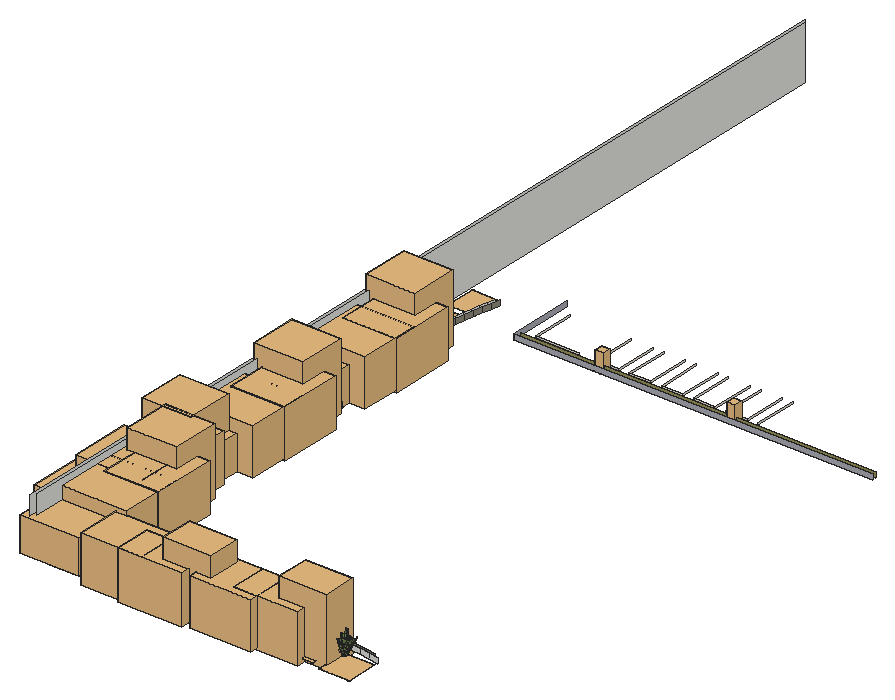
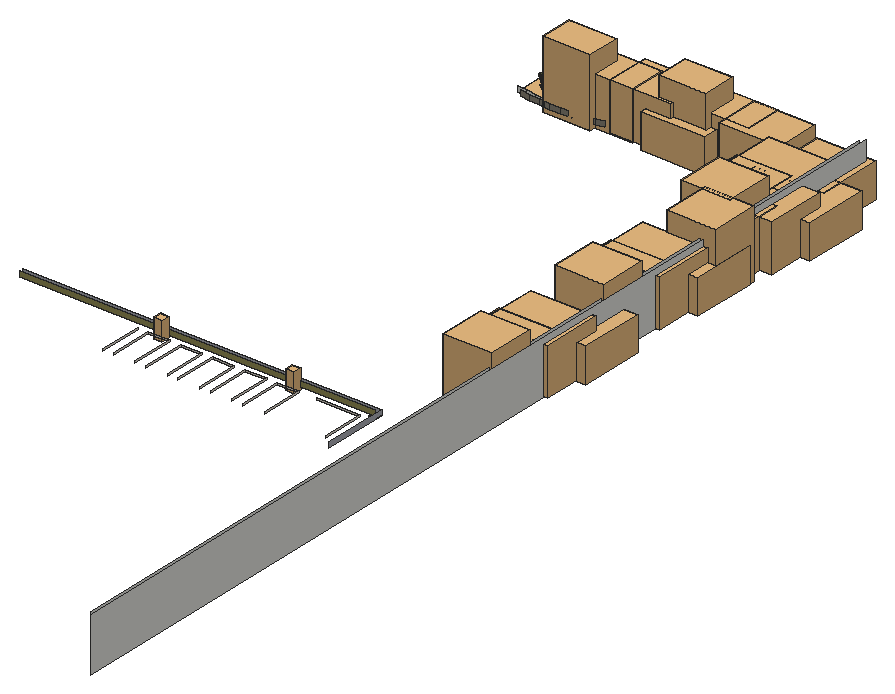
# SketchUp Ruby script. Lengths in inches.
U = 1.inch
M = Sketchup.active_model
def pt(a) = Geom::Point3d.new(a.map { |v| v * U })
def face(e, loops, mat)
  f = e.add_face(loops[0].map { |a| pt(a) })
  loops[1..].each { |l| e.add_face(l.map { |a| pt(a) }).erase! }
  f.material = f.back_material = mat if mat
  f
end
# faces: each face lists its corners as indices into pts; further lists are holes
def faces(e, pts, list, mat = nil) = list.each { |f| face(e, (f[0].is_a?(Array) ? f : [f]).map { |l| l.map { |i| pts[i] } }, mat) }
# xy, xz, yz: faces in a plane at the given z, y or x. An outline is a flat list of corners, or four numbers for a rectangle; further outlines are holes
def ring(l) = l.size == 4 ? [[l[0], l[1]], [l[2], l[1]], [l[2], l[3]], [l[0], l[3]]] : l.each_slice(2).to_a
def flat(e, list, mat, &to3) = list.each { |f| face(e, (f[0].is_a?(Array) ? f : [f]).map { |l| ring(l).map { |u, v| to3.(u, v) } }, mat) }
def xy(e, z, list, mat = nil) = flat(e, list, mat) { |x, y| [x, y, z] }
def xz(e, y, list, mat = nil) = flat(e, list, mat) { |x, z| [x, y, z] }
def yz(e, x, list, mat = nil) = flat(e, list, mat) { |y, z| [x, y, z] }
def lines(e, pts, list) = list.each { |a, b| e.add_line(pt(pts[a]), pt(pts[b])) }
# prism: a flat outline (further loops are holes) pulled along v
def prism(e, loops, v, mat = nil)
  f = face(e, loops, mat); d = Geom::Vector3d.new(v.map { |x| x * U })
  f.pushpull(f.normal.samedirection?(d) ? d.length : -d.length)
end
def box(e, o, s, mat = nil) = prism(e, [[o, [o[0] + s[0], o[1], o[2]], [o[0] + s[0], o[1] + s[1], o[2]], [o[0], o[1] + s[1], o[2]]]], [0, 0, s[2]], mat)
def at(x, y, z, deg = 0) = Geom::Transformation.translation(pt([x, y, z])) * Geom::Transformation.rotation(ORIGIN, Z_AXIS, deg.degrees)
def axes(o, x, y, z) = Geom::Transformation.new([*x, 0, *y, 0, *z, 0, *pt(o).to_a, 1])
def part(name) = M.definitions.add(name)
# library, detail: a bought-in or finely detailed component or shape, given as its bounding box
def library(name, o, s) = part(name).tap { |d| box(d.entities, o, s) }
def detail(e, o, s) = box(e.add_group.entities, o, s)
def put(e, d, t, mat = nil) = e.add_instance(d, t).tap { |i| i.material = mat if mat }
def group(e, t, mat = nil) = e.add_group.tap { |g| g.transformation = t; g.material = mat if mat }.entities
root = M.entities
M.materials.add("Marble_01_1K").color = [230, 221, 211]
M.materials.add("Marble_20_1K").color = [172, 173, 182]
M.materials.add("Material__4").color = [36, 36, 36]
M.materials.add("Material__6").color = [79, 108, 5]
M.materials.add("Plaster_06_1K").color = [141, 135, 122]
M.materials.add("Soil_04_1K").color = [152, 146, 88]
M.materials.add("calathea lutea").color = [121, 145, 80]
c1 = library("ew",[-14.92,-16.84,0],[29.84,33.68,0.01])
c2 = library("t1",[-17.79,-17.21,0],[35.58,34.42,0.01])
c3 = library("tt",[-12.4,-12.1,0],[24.8,24.2,0.01])
c4 = part("Group\#156")
g1 = group(c4.entities,at(8.61,38.85,0))
xy(g1,0,[[0,0,2.82,19.1,22.58,0],[22.58,0,2.82,19.1,22.58,19.1]],"calathea lutea")
p = [[2.82,19.1,0],[7.19,48.22,5.13],[10.77,48.22,5.13],[12.74,48.22,5.13],[22.58,48.22,5.13],[22.58,19.1,0]]
faces(g1,p,[[0,1,2,3,4,5]],"calathea lutea")
g2 = group(c4.entities,at(-0.77,-7.77,0))
p = [[14.8125,23.31,1.46],[21.35,23.31,0],[14.8125,0,1.46],[21.35,0,0],[27.89,0,1.46],[27.89,23.31,1.46],
  [8.27,46.62,2.92],[21.35,46.62,0],[34.4375,46.62,2.92],[4.47,23.31,6.43],[0,0,8.59],[33.76,0,4.28],
  [33.76,23.31,4.28]]
faces(g2,p,[[0,1,2],[3,2,1],[4,3,5],[1,5,3],[6,7,0],[1,0,7],[5,1,8],[7,8,1],
  [9,0,2,10],[11,4,5,12],[9,6,0],[12,5,8]],"calathea lutea")
c5 = part("Group\#150")
xy(c5.entities,0,[[0,0,0,33.87,27.21,33.87,19.71,0]],"calathea lutea")
c6 = part("Group\#157")
xy(c6.entities,1.04,[[21.13,33.87,21.13,57.59,32.375,57.59,27.12,33.87]],"calathea lutea")
xy(c6.entities,1.32,[[0.12,33.87,7.74,57.59]],"calathea lutea")
p = [[7.74,33.87,1.32],[11.8,57.59,0.61],[15.24,57.59,0],[15.24,33.87,0],[18.43,57.59,0.5625],[21.13,57.59,1.04],
  [21.13,33.87,1.04],[15.24,77.7,2.36],[21.13,77.7,3.4],[7.74,57.59,1.32],[7.74,77.7,3.69],[36.83,77.7,3.4],
  [32.375,57.59,1.04],[0.12,57.59,1.32],[0.12,77.7,3.69]]
faces(c6.entities,p,[[0,1,2,3],[3,2,4],[3,4,5,6],[7,2,1],[8,4,2,7],[0,9,1],[7,1,9,10],[8,5,4],
  [11,12,5,8],[10,9,13,14]],"calathea lutea")
put(c6.entities,c5,axes([0,-16.9375,0],[1,0,0],[0,1.5,0],[0,0,1]))
c7 = part("Group\#155")
g3 = group(c7.entities,at(0,-17.3,0))
xy(g3,0,[[0,0,28.07,51.9]],"calathea lutea")
g4 = group(c7.entities,at(0.9,34.6,0))
xy(g4,0,[[13.14,0,13.14,26.22,16.85,26.22],[13.14,0,16.85,26.22,20.16,26.22,20.16,0]],"calathea lutea")
p = [[6.36,0,1.82],[9.95,26.22,0.86],[13.14,26.22,0],[13.14,0,0],[20.16,0,0],[20.16,26.22,0],
  [27.07,26.22,1.22],[27.07,0,1.22],[13.14,49.5625,5.91],[20.16,49.5625,5.91],[16.85,26.22,0],[27.07,49.5625,7.125],
  [6.36,26.22,1.82],[6.36,49.5625,7.72],[0,0,4.78],[0,26.22,4.78],[0,49.5625,10.6875]]
faces(g4,p,[[0,1,2,3],[4,5,6,7],[8,2,1],[9,10,2,8],[9,5,10],[11,6,5,9],[0,12,1],[8,1,12,13],
  [14,15,12,0],[13,12,15,16]],"calathea lutea")
c8 = part("Group\#154")
put(c8.entities,c5,axes([0,-16.9375,0],[1,0,0],[0,1.5,0],[0,0,1]))
g5 = group(c8.entities,at(-0.23,33.4,-0.35))
p = [[15.12,39.14,-19.87],[15.12,20.54,-11.86],[11.68,20.84,-11.33],[21.02,39.66,-18.97],[18.3125,20.82,-11.37],[7.62,21.2,-10.71],
  [7.62,39.8,-18.72],[21.02,21.06,-10.96],[36.72,39.66,-18.97],[32.26,21.06,-10.96],[0,21.2,-10.71],[0,39.8,-18.72],
  [7.62,0.66,1.15],[15.12,0,0],[21.02,0.52,0.9],[27.01,0.52,0.9],[0,0.66,1.15]]
faces(g5,p,[[0,1,2],[3,4,1,0],[0,2,5,6],[3,7,4],[8,9,7,3],[6,5,10,11],[12,2,1,13],[13,1,4],
  [13,4,7,14],[12,5,2],[14,7,9,15],[16,10,5,12]],"calathea lutea")
c9 = part("Foliage cluster")
put(c9.entities,c4,axes([37.24,8.07,75.17],[1,0,0],[0,0.45554,-0.89021],[0,0.89021,0.45554]))
put(c9.entities,c6,axes([69.44,65.48,16.68],[-0.53288,-0.84619,0],[0.14694,-0.09253,0.98481],[-0.83334,0.52478,0.17365]))
put(c9.entities,c7,axes([47.9375,70.43,17.04],[0.74664,-0.66523,0],[0.11552,0.12965,0.98481],[-0.65512,-0.7353,0.17365]))
put(c9.entities,c4,axes([76.19,10.66,75.17],[0.70711,0.70711,0],[-0.32212,0.32212,-0.89021],[-0.62948,0.62948,0.45554]))
put(c9.entities,c4,axes([101.91,40.03,75.17],[0,1,0],[-0.45554,0,-0.89021],[-0.89021,0,0.45554]))
put(c9.entities,c4,axes([99.32,78.99,75.17],[-0.70711,0.70711,0],[-0.32212,-0.32212,-0.89021],[-0.62948,-0.62948,0.45554]))
put(c9.entities,c7,axes([34.81,63.36,17.04],[0.99956,-0.02967,0],[0.00515,0.17357,0.98481],[-0.02922,-0.98437,0.17365]))
put(c9.entities,c7,axes([48,37.4,15.8],[-0.14436,0.98953,0],[-0.40248,-0.05871,0.91355],[0.90398,0.13188,0.40674]))
put(c9.entities,c6,axes([56.87,39.77,12.28],[-0.67695,0.4263,0],[-0.18016,-0.28609,0.72505],[0.38636,0.61353,0.33809]))
put(c9.entities,c6,axes([36.12,43.25,12.28],[0.18947,0.77724,0],[-0.32848,0.08007,0.72505],[0.70442,-0.17172,0.33809]))
put(c9.entities,c8,axes([35.1,54.93,11.375],[0.79719,0.06694,0],[-0.03636,0.43302,0.6717],[0.05621,-0.66934,0.43454]))
put(c9.entities,c6,axes([41.66,47.32,12.28],[0.45082,0.66088,0],[-0.2793,0.19053,0.72505],[0.59896,-0.40858,0.33809]))
put(c9.entities,c6,axes([47.89,59.4,12.28],[0.79719,0.06694,0],[-0.02829,0.33691,0.72505],[0.06067,-0.7225,0.33809]))
put(c9.entities,c8,axes([29.53,49.96,11.375],[0.65692,0.45657,0],[-0.248,0.35682,0.6717],[0.38335,-0.55156,0.43454]))
put(c9.entities,c8,axes([29.9,49.27,12.86],[0.34062,0.72386,0],[-0.22849,0.10752,0.7591],[0.68685,-0.32321,0.25252]))
put(c9.entities,c8,axes([36.33,48.82,8.99],[0.09232,0.62522,0],[-0.3396,0.05015,0.53064],[0.52495,-0.07752,0.34329]))
put(c9.entities,c8,axes([49.82,38.52,8.99],[-0.54622,0.31791,0],[-0.17268,-0.29669,0.53064],[0.26692,0.45862,0.34329]))
put(c9.entities,c8,axes([55.68,39.21,8.99],[-0.632,0.00221,0],[-0.0012,-0.34328,0.53064],[0.00185,0.53064,0.34329]))
c10 = library("Group\#28",[0,0,0],[86.94,78.77,46.4375])
c11 = library("Group\#14",[-978.71,-103.24,719.12],[90.2,76.4,68.29])
c12 = library("Group\#13",[-906.16,-138.28,686.8],[98.25,106.18,75.79])
c13 = library("Group\#202",[-3.47,-2.45,12.47],[53.14,54.93,75.51])
c14 = part("Group\#41")
put(c14.entities,c9,axes([161.54,64.35,6.01],[0.19523,-0.19694,0],[0.19694,0.19523,0],[0,0,0.24957]))
put(c14.entities,c10,axes([0,37.34,0.92],[0.83,0,0],[0,0.83,0],[0,0,0.83]))
put(c14.entities,c11,axes([859.63,98.87,-568.1],[0.79,0,0],[0,0.79,0],[0,0,0.79]),"Material__4")
put(c14.entities,c12,axes([669.69,114.28,-472.48],[0.69,0,0],[0,0.69,0],[0,0,0.69]),"Material__6")
put(c14.entities,c13,at(132.78,33.9375,-12.6))
c15 = library("light",[-4,-4,0],[8,8,0.01])
c16 = library("Group\#54",[0,0,0],[2062.46,2062.46,4833.66])
c17 = part("Landscape+Light")
put(c17.entities,c16,at(-2096.57,-1031.23,-3775.98))
xz(root,562.78,[[98.71,0,498.69,6]],"Marble_20_1K")
xz(root,567.28,[[103.21,0,498.69,6]],"Soil_04_1K")
xz(root,576.64,[[180.08,0,204.08,2],[216.08,0,240.08,2],[252.08,0,276.08,2],[288.08,0,312.08,2],[324.08,0,348.08,2]],"Marble_01_1K")
xz(root,576.78,[[111.43,0,159.43,2]],"Marble_01_1K")
yz(root,8.46,[[0.95,0,1080.74,60]])
yz(root,12.46,[[4.95,0,1076.74,60]])
yz(root,98.71,[[562.78,0,636.6,6]],"Marble_20_1K")
yz(root,111.43,[[576.78,0,624.64,2]],"Marble_01_1K")
yz(root,180.08,[[576.64,0,624.64,2]],"Marble_01_1K")
yz(root,204.08,[[576.64,0,624.64,2]],"Marble_01_1K")
yz(root,216.08,[[576.64,0,624.64,2]],"Marble_01_1K")
yz(root,240.08,[[576.64,0,624.64,2]],"Marble_01_1K")
yz(root,252.08,[[576.64,0,624.64,2]],"Marble_01_1K")
yz(root,276.08,[[576.64,0,624.64,2]],"Marble_01_1K")
yz(root,288.08,[[576.64,0,624.64,2]],"Marble_01_1K")
yz(root,312.08,[[576.64,0,624.64,2]],"Marble_01_1K")
yz(root,324.08,[[576.64,0,624.64,2]],"Marble_01_1K")
yz(root,348.08,[[576.64,0,624.64,2]],"Marble_01_1K")
yz(root,360.08,[[576.64,0,624.64,2]],"Marble_01_1K")
p = [[183.9,25.07,0],[194.74,24.51,0],[194.74,24.51,6],[183.9,25.07,6],[205.71,25.03,0],[205.71,25.03,6],
  [216.79,26.42,0],[216.79,26.42,6],[173.26,26.9,0],[173.26,26.9,6],[227.98,28.46,0],[227.98,28.46,6],
  [162.9,29.8,0],[162.9,29.8,6],[195.48,27.51,0],[184.7,28,0],[184.7,28,6],[195.48,27.51,6],
  [206.47,28.12,0],[206.47,28.12,6],[174.14,29.78,0],[174.14,29.78,6],[217.65,29.59,0],[217.65,29.59,6],
  [239.25,30.9375,0],[239.25,30.9375,6],[229,31.73,0],[229,31.73,6],[152.68,33.2,0],[152.68,33.2,6],
  [163.75,32.68,0],[163.75,32.68,6],[250.61,33.66,0],[250.61,33.66,6],[240.5,34.3125,0],[240.5,34.3125,6],
  [153.33,36.15,0],[153.33,36.15,6],[36.37,33.08,0],[45.35,34.71,0],[45.35,34.71,6],[36.37,33.08,6],
  [37.51,35.49,0],[37.51,35.49,6],[142.43,36.56,0],[142.43,36.56,6],[262.02,36.42,0],[262.02,36.42,6],
  [252.13,37.12,0],[252.13,37.12,6],[54.59,36.375,0],[54.59,36.375,6],[38.66,37.9,0],[38.66,37.9,6],
  [142.71,39.61,0],[142.71,39.61,6],[64.7,38.09,0],[64.7,38.09,6],[273.48,39.01,0],[273.48,39.01,6],
  [131.97,39.34,0],[131.97,39.34,6],[51.57,38.89,0],[41.67,37.13,0],[41.67,37.13,6],[51.57,38.89,6],
  [43.09,40.39,0],[43.09,40.39,6],[263.875,39.93,0],[263.875,39.93,6],[39.81,40.34,0],[39.81,40.34,6],
  [75.5,39.68,0],[75.5,39.68,6],[61.79,40.65,0],[61.79,40.65,6],[284.95,41.24,0],[284.95,41.24,6],
  [121.11,41.12,0],[121.11,41.12,6],[354.15,41.14,0],[365.76,39.31,0],[365.76,39.31,6],[354.15,41.14,6],
  [131.72,42.47,0],[131.72,42.47,6],[86.77,40.96,0],[86.77,40.96,6],[275.71,42.54,0],[275.71,42.54,6],
  [41,43.32,0],[41,43.32,6],[44.54,44.33,0],[44.54,44.33,6],[72.8,42.34,0],[72.8,42.34,6],
  [98.28,41.75,0],[98.28,41.75,6],[109.81,41.86,0],[109.81,41.86,6],[342.54,42.61,0],[342.54,42.61,6],
  [296.43,42.92,0],[296.43,42.92,6],[84.39,43.75,0],[84.39,43.75,6],[120.22,44.23,0],[120.22,44.23,6],
  [287.6,44.73,0],[287.6,44.73,6],[330.96,43.62,0],[330.96,43.62,6],[307.9,43.87,0],[307.9,43.87,6],
  [42.25,47.02,0],[42.25,47.02,6],[359.53,43.37,0],[347.53,45.05,0],[347.53,45.05,6],[359.53,43.37,6],
  [319.41,44.07,0],[319.41,44.07,6],[96.32,44.66,0],[96.32,44.66,6],[108.34,44.89,0],[108.34,44.89,6],
  [46,49.13,0],[46,49.13,6],[299.55,46.27,0],[299.55,46.27,6],[335.52,46.29,0],[335.52,46.29,6],
  [311.53,47.01,0],[311.53,47.01,6],[323.52,46.98,0],[323.52,46.98,6],[43.53,51.45,0],[43.53,51.45,6],
  [47.49,54.8125,0],[47.49,54.8125,6],[44.84,56.61,0],[44.84,56.61,6],[48.99,61.4,0],[48.99,61.4,6],
  [46.16,62.5,0],[46.16,62.5,6],[50.52,68.9,0],[50.52,68.9,6],[47.51,69.13,0],[47.51,69.13,6],
  [52.08,77.33,0],[52.08,77.33,6],[48.88,76.51,0],[48.88,76.51,6],[50.3125,84.62,0],[50.3125,84.62,6],
  [53.7,86.63,0],[53.7,86.63,6],[51.73,93.31,0],[51.73,93.31,6],[55.27,96.65,0],[55.27,96.65,6],
  [53.03,102.4375,0],[53.03,102.4375,6],[56.63,107.19,0],[56.63,107.19,6],[54.11,111.88,0],[54.11,111.88,6],
  [57.64,118.07,0],[57.64,118.07,6],[54.85,121.51,0],[54.85,121.51,6],[58.12,129.1,0],[58.12,129.1,6],
  [55.14,131.18,0],[55.14,131.18,6],[57.92,140.1,0],[57.92,140.1,6],[54.88,140.77,0],[54.88,140.77,6],
  [56.89,150.88,0],[56.89,150.88,6],[53.96,150.125,0],[53.96,150.125,6],[52.3,159.14,0],[52.3,159.14,6],
  [54.875,161.27,0],[54.875,161.27,6],[49.9375,167.89,0],[49.9375,167.89,6],[52.04,171.24,0],[52.04,171.24,6],
  [47.16,176.49,0],[47.16,176.49,6],[48.82,180.9375,0],[48.82,180.9375,6],[44.27,185.04,0],[44.27,185.04,6],
  [45.66,190.49,0],[45.66,190.49,6],[41.59,193.65,0],[41.59,193.65,6],[43.02,200.04,0],[43.02,200.04,6],
  [39.4375,202.41,0],[39.4375,202.41,6],[41.33,209.72,0],[41.33,209.72,6],[38.14,211.375,0],[38.14,211.375,6],
  [40.74,219.59,0],[40.74,219.59,6],[37.73,220.46,0],[37.73,220.46,6],[41.1,229.64,0],[41.1,229.64,6],
  [38.09,229.64,0],[38.09,229.64,6],[39.08,238.9,0],[39.08,238.9,6],[42.24,239.85,0],[42.24,239.85,6],
  [40.58,248.23,0],[40.58,248.23,6],[44,250.22,0],[44,250.22,6],[42.46,257.64,0],[42.46,257.64,6],
  [46.21,260.72,0],[46.21,260.72,6],[44.61,267.1,0],[44.61,267.1,6],[48.7,271.34,0],[48.7,271.34,6],
  [46.9,276.62,0],[46.9,276.62,6],[51.3,282.06,0],[51.3,282.06,6],[49.21,286.18,0],[49.21,286.18,6],
  [53.86,292.86,0],[53.86,292.86,6],[51.43,295.76,0],[51.43,295.76,6],[56.18,303.74,0],[56.18,303.74,6],
  [53.45,305.375,0],[53.45,305.375,6],[58.125,314.67,0],[58.125,314.67,6],[55.14,314.99,0],[55.14,314.99,6],
  [59.51,325.64,0],[59.51,325.64,6],[56.39,324.6,0],[56.39,324.6,6],[57.11,334.21,0],[57.11,334.21,6],
  [60.21,336.63,0],[60.21,336.63,6],[57.31,343.85,0],[57.31,343.85,6],[60.26,347.64,0],[60.26,347.64,6],
  [57.04,353.52,0],[57.04,353.52,6],[59.73,358.66,0],[59.73,358.66,6],[56.36,363.22,0],[56.36,363.22,6],
  [58.73,369.68,0],[58.73,369.68,6],[55.33,372.93,0],[55.33,372.93,6],[57.3125,380.7,0],[57.3125,380.7,6],
  [53.99,382.65,0],[53.99,382.65,6],[55.58,391.71,0],[55.58,391.71,6],[52.42,392.38,0],[52.42,392.38,6],
  [53.61,402.7,0],[53.61,402.7,6],[50.66,402.12,0],[50.66,402.12,6],[48.78,411.85,0],[48.78,411.85,6],
  [51.48,413.66,0],[51.48,413.66,6],[46.83,421.58,0],[46.83,421.58,6],[49.28,424.6,0],[49.28,424.6,6],
  [44.87,431.29,0],[44.87,431.29,6],[47.09,435.5,0],[47.09,435.5,6],[42.96,440.99,0],[42.96,440.99,6],
  [45,446.36,0],[45,446.36,6],[41.16,450.67,0],[41.16,450.67,6],[43.08,457.16,0],[43.08,457.16,6],
  [39.52,460.32,0],[39.52,460.32,6],[41.42,467.91,0],[41.42,467.91,6],[38.11,469.95,0],[38.11,469.95,6],
  [40.1,478.6,0],[40.1,478.6,6],[36.98,479.55,0],[36.98,479.55,6],[39.2,489.21,0],[39.2,489.21,6],
  [36.2,489.1,0],[36.2,489.1,6],[35.8,498.61,0],[35.8,498.61,6],[38.78,499.75,0],[38.78,499.75,6],
  [35.75,508.04,0],[35.75,508.04,6],[38.79,510.22,0],[38.79,510.22,6],[36.03,517.42,0],[36.03,517.42,6],
  [39.2,520.63,0],[39.2,520.63,6],[36.6,526.74,0],[36.6,526.74,6],[39.97,530.98,0],[39.97,530.98,6],
  [37.4375,536.01,0],[37.4375,536.01,6],[41.04,541.28,0],[41.04,541.28,6],[38.51,545.22,0],[38.51,545.22,6],
  [42.39,551.52,0],[42.39,551.52,6],[39.78,554.39,0],[39.78,554.39,6],[43.96,561.72,0],[43.96,561.72,6],
  [41.22,563.51,0],[41.22,563.51,6],[45.72,571.88,0],[45.72,571.88,6],[42.8,572.6,0],[42.8,572.6,6],
  [47.61,582.01,0],[47.61,582.01,6],[44.49,581.64,0],[44.49,581.64,6],[46.26,590.66,0],[46.26,590.66,6],
  [49.61,592.11,0],[49.61,592.11,6],[48.07,599.64,0],[48.07,599.64,6],[51.66,602.1875,0],[51.66,602.1875,6]]
faces(root,p,[[0,1,2,3],[1,4,5,2],[4,6,7,5],[8,0,3,9],[6,10,11,7],[12,8,9,13],[10,24,25,11],[28,12,13,29],
  [24,32,33,25],[38,39,40,41],[42,38,41,43],[44,28,29,45],[32,46,47,33],[39,50,51,40],[52,42,43,53],[50,56,57,51],
  [46,58,59,47],[60,44,45,61],[70,52,53,71],[56,72,73,57],[58,76,77,59],[78,60,61,79],[80,81,82,83],[72,86,87,73],
  [90,70,71,91],[86,96,97,87],[98,78,79,99],[100,80,83,101],[76,102,103,77],[96,98,99,97],[110,100,101,111],[102,112,113,103],
  [114,90,91,115],[120,110,111,121],[112,120,121,113],[136,114,115,137],[140,136,137,141],[144,140,141,145],[148,144,145,149],[152,148,149,153],
  [154,152,153,155],[158,154,155,159],[162,158,159,163],[166,162,163,167],[170,166,167,171],[174,170,171,175],[178,174,175,179],[182,178,179,183],
  [184,182,183,185],[188,184,185,189],[192,188,189,193],[196,192,193,197],[200,196,197,201],[204,200,201,205],[208,204,205,209],[212,208,209,213],
  [216,212,213,217],[218,216,217,219],[222,218,219,223],[226,222,223,227],[230,226,227,231],[234,230,231,235],[238,234,235,239],[242,238,239,243],
  [246,242,243,247],[250,246,247,251],[254,250,251,255],[256,254,255,257],[260,256,257,261],[264,260,261,265],[268,264,265,269],[272,268,269,273],
  [276,272,273,277],[280,276,277,281],[284,280,281,285],[286,284,285,287],[290,286,287,291],[294,290,291,295],[298,294,295,299],[302,298,299,303],
  [306,302,303,307],[310,306,307,311],[314,310,311,315],[318,314,315,319],[320,318,319,321],[324,320,321,325],[328,324,325,329],[332,328,329,333],
  [336,332,333,337],[340,336,337,341],[344,340,341,345],[348,344,345,349],[352,348,349,353],[356,352,353,357],[358,356,357,359],[362,358,359,363]])
faces(root,p,[[14,15,16,17],[18,14,17,19],[15,20,21,16],[22,18,19,23],[26,22,23,27],[20,30,31,21],[34,26,27,35],[30,36,37,31],
  [48,34,35,49],[36,54,55,37],[62,63,64,65],[63,66,67,64],[68,48,49,69],[74,62,65,75],[54,84,85,55],[88,68,69,89],
  [66,92,93,67],[94,74,75,95],[104,94,95,105],[84,106,107,85],[108,88,89,109],[116,117,118,119],[122,104,105,123],[106,124,125,107],
  [92,126,127,93],[124,122,123,125],[128,108,109,129],[117,130,131,118],[132,128,129,133],[130,134,135,131],[134,132,133,135],[126,138,139,127],
  [138,142,143,139],[142,146,147,143],[146,150,151,147],[150,156,157,151],[156,160,161,157],[160,164,165,161],[164,168,169,165],[168,172,173,169],
  [172,176,177,173],[176,180,181,177],[180,186,187,181],[186,190,191,187],[190,194,195,191],[194,198,199,195],[198,202,203,199],[202,206,207,203],
  [206,210,211,207],[210,214,215,211],[214,220,221,215],[220,224,225,221],[224,228,229,225],[228,232,233,229],[232,236,237,233],[236,240,241,237],
  [240,244,245,241],[244,248,249,245],[248,252,253,249],[252,258,259,253],[258,262,263,259],[262,266,267,263],[266,270,271,267],[270,274,275,271],
  [274,278,279,275],[278,282,283,279],[282,288,289,283],[288,292,293,289],[292,296,297,293],[296,300,301,297],[300,304,305,301],[304,308,309,305],
  [308,312,313,309],[312,316,317,313],[316,322,323,317],[322,326,327,323],[326,330,331,327],[330,334,335,331],[334,338,339,335],[338,342,343,339],
  [342,346,347,343],[346,350,351,347],[350,354,355,351],[354,360,361,355],[360,364,365,361]],"Plaster_06_1K")
put(root,c1,at(30.54,17.9375,0,180))
put(root,c2,axes([125.77,17.9375,0],[0,-1,0],[-1,0,0],[0,0,1]))
put(root,c2,axes([227.66,17.9375,0],[0,-1,0],[-1,0,0],[0,0,1]))
put(root,c2,axes([348.22,17.9375,0],[0,-1,0],[-1,0,0],[0,0,1]))
put(root,c3,axes([45.09,18.42,0],[0,-1,0],[-1,0,0],[0,0,1]))
put(root,c3,axes([146.98,18.42,0],[0,-1,0],[-1,0,0],[0,0,1]))
put(root,c3,axes([267.54,18.42,0],[0,-1,0],[-1,0,0],[0,0,1]))
put(root,c14,axes([28.13,-21.13,-5.25],[1,0,0],[0,0.67442,0],[0,0,1]))
g6 = group(root,at(149.82,-21.13,-5.25))
put(g6,c9,axes([161.54,52.83,6.01],[0.19523,-0.13282,0],[0.19694,0.13166,0],[0,0,0.24957]))
put(g6,c10,axes([0,25.1875,0.92],[0.83,0,0],[0,0.55977,0],[0,0,0.83]))
put(g6,c11,axes([859.63,76.11,-568.1],[0.79,0,0],[0,0.53279,0],[0,0,0.79]),"Material__4")
put(g6,c12,axes([669.69,77.07,-472.48],[0.69,0,0],[0,0.46535,0],[0,0,0.69]),"Material__6")
put(g6,c13,axes([132.78,32.32,-12.6],[1,0,0],[0,0.67442,0],[0,0,1]))
put(root,c1,axes([81.53,20.08,0],[0,-1,0],[-1,0,0],[0,0,1]))
put(root,c1,axes([183.42,20.08,0],[0,-1,0],[-1,0,0],[0,0,1]))
put(root,c1,axes([303.98,20.08,0],[0,-1,0],[-1,0,0],[0,0,1]))
put(root,c2,at(28.39,62.18,0,180))
put(root,c3,at(28.88,92.72,0,180))
put(root,c14,at(103.85,-3.91,0.12,90))
put(root,c1,at(30.54,129.16,0,180))
put(root,c14,at(80.46,45.39,0.12,90))
put(root,c2,at(28.39,173.4,0,180))
put(root,c3,at(28.88,194.52,0,180))
put(root,c1,at(30.54,230.96,0,180))
put(root,c2,at(28.39,275.2,0,180))
put(root,c14,at(95.48,182.65,0.12,90))
put(root,c3,at(28.88,315.08,0,180))
put(root,c1,at(30.54,351.51,0,180))
put(root,c2,at(28.39,395.75,0,180))
put(root,c3,at(28.88,433.12,0,180))
put(root,c14,at(95.48,338.78,0.12,90))
put(root,c1,at(30.54,469.56,0,180))
put(root,c2,at(28.39,513.8,0,180))
put(root,c3,at(28.88,555.46,0,180))
put(root,c15,at(102.52,566.89,0))
put(root,c15,at(192.08,566.89,0))
put(root,c17,axes([185.79,571.62,13.79],[-0.0044,0,0],[0,-0.0044,0],[0,0,0.0044]))
put(root,c17,axes([332.82,571.62,13.79],[-0.0044,0,0],[0,-0.0044,0],[0,0,0.0044]))
put(root,c1,at(30.54,591.9,0,180))
